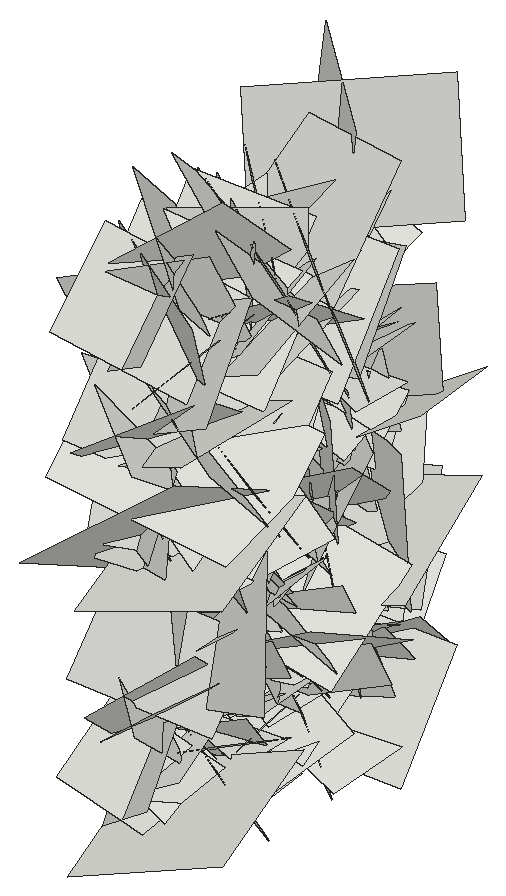
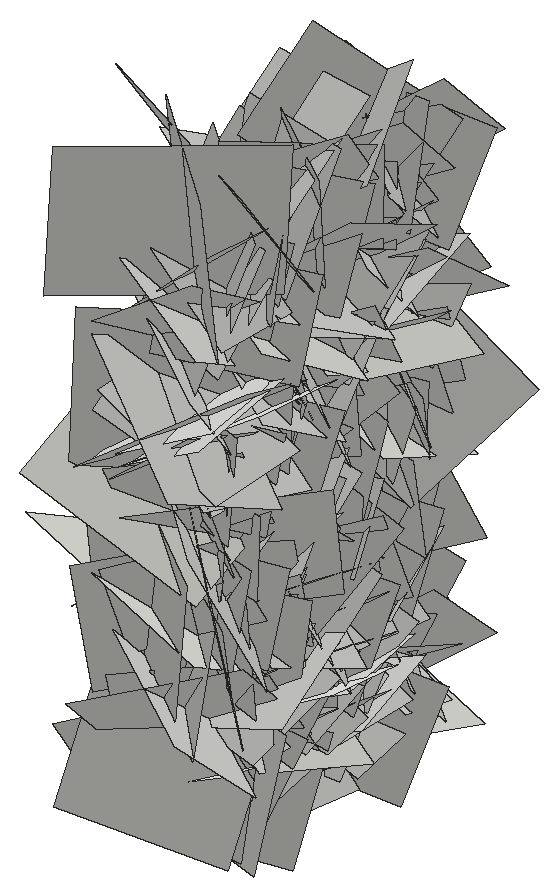
# SketchUp Ruby script. Lengths in inches.
U = 1.inch
M = Sketchup.active_model
def pt(a) = Geom::Point3d.new(a.map { |v| v * U })
def face(e, loops, mat)
  f = e.add_face(loops[0].map { |a| pt(a) })
  loops[1..].each { |l| e.add_face(l.map { |a| pt(a) }).erase! }
  f.material = f.back_material = mat if mat
  f
end
# faces: each face lists its corners as indices into pts; further lists are holes
def faces(e, pts, list, mat = nil) = list.each { |f| face(e, (f[0].is_a?(Array) ? f : [f]).map { |l| l.map { |i| pts[i] } }, mat) }
# xy, xz, yz: faces in a plane at the given z, y or x. An outline is a flat list of corners, or four numbers for a rectangle; further outlines are holes
def ring(l) = l.size == 4 ? [[l[0], l[1]], [l[2], l[1]], [l[2], l[3]], [l[0], l[3]]] : l.each_slice(2).to_a
def flat(e, list, mat, &to3) = list.each { |f| face(e, (f[0].is_a?(Array) ? f : [f]).map { |l| ring(l).map { |u, v| to3.(u, v) } }, mat) }
def xy(e, z, list, mat = nil) = flat(e, list, mat) { |x, y| [x, y, z] }
def xz(e, y, list, mat = nil) = flat(e, list, mat) { |x, z| [x, y, z] }
def yz(e, x, list, mat = nil) = flat(e, list, mat) { |y, z| [x, y, z] }
def lines(e, pts, list) = list.each { |a, b| e.add_line(pt(pts[a]), pt(pts[b])) }
# prism: a flat outline (further loops are holes) pulled along v
def prism(e, loops, v, mat = nil)
  f = face(e, loops, mat); d = Geom::Vector3d.new(v.map { |x| x * U })
  f.pushpull(f.normal.samedirection?(d) ? d.length : -d.length)
end
def box(e, o, s, mat = nil) = prism(e, [[o, [o[0] + s[0], o[1], o[2]], [o[0] + s[0], o[1] + s[1], o[2]], [o[0], o[1] + s[1], o[2]]]], [0, 0, s[2]], mat)
def at(x, y, z, deg = 0) = Geom::Transformation.translation(pt([x, y, z])) * Geom::Transformation.rotation(ORIGIN, Z_AXIS, deg.degrees)
def axes(o, x, y, z) = Geom::Transformation.new([*x, 0, *y, 0, *z, 0, *pt(o).to_a, 1])
def part(name) = M.definitions.add(name)
# library, detail: a bought-in or finely detailed component or shape, given as its bounding box
def library(name, o, s) = part(name).tap { |d| box(d.entities, o, s) }
def detail(e, o, s) = box(e.add_group.entities, o, s)
def put(e, d, t, mat = nil) = e.add_instance(d, t).tap { |i| i.material = mat if mat }
def group(e, t, mat = nil) = e.add_group.tap { |g| g.transformation = t; g.material = mat if mat }.entities
root = M.entities
c1 = part("Component\#6")
p = [[0.01,0,0],[0,3.24,4.54],[4.32,3.24,4.54],[4.33,0,0]]
faces(c1.entities,p,[[0,1,2,3]])
put(root,c1,axes([424.49,166.18,19.56],[0.12535,0.0531,1.28965],[0.2192,1.27754,-0.07157],[-1.35051,0.21229,0.10808]))
put(root,c1,axes([424.49,167.01,8.33],[-0.18631,0.3359,0.73427],[-0.04897,0.74605,-0.35235],[-0.8545,-0.11599,-0.1399]))
put(root,c1,axes([420.52,159.82,10.86],[-0.164,0.05549,-0.7166],[0.119,-0.72215,-0.08015],[0.75252,0.12629,-0.14349]))
put(root,c1,axes([424.49,164.72,6.23],[0.02586,0.29335,1.1723],[0.23754,1.1511,-0.29271],[-1.25874,0.22326,-0.03115]))
put(root,c1,axes([420.52,164.71,11.17],[-0.09162,-0.23701,0.75882],[-0.09076,0.76162,0.22813],[0.83777,0.05659,0.1077]))
put(root,c1,axes([420.52,167.39,12.19],[-0.06725,0.11282,-0.6237],[0.12717,-0.61335,-0.12315],[0.65971,0.12973,-0.03984]))
put(root,c1,axes([420.52,158.25,7.85],[0.01053,0.60228,-0.51533],[-0.19634,-0.49934,-0.58716],[0.81696,-0.12777,-0.13447]))
put(root,c1,axes([424.49,165.51,17.74],[-0.00528,-0.97827,-0.44464],[0.11526,-0.44282,0.97306],[-1.13321,-0.04048,0.10104]))
put(root,c1,axes([424.49,165.75,-1.09],[0.03685,-0.4153,0.96157],[0.02645,0.96216,0.41465],[-1.10996,0.00914,0.04181]))
put(root,c1,axes([424.49,167.74,3.51],[0.11337,-0.86322,0.3774],[-0.28126,0.33685,0.84566],[-0.95821,-0.201,-0.20357]))
put(root,c1,axes([424.49,161.03,4.22],[-0.00206,0.54706,-0.73945],[-0.10036,-0.73565,-0.544],[-0.96983,0.07497,0.05787]))
put(root,c1,axes([424.49,158.84,13.7],[-0.15038,-0.75335,0.50607],[0.08727,0.49942,0.76653],[-0.95804,0.16374,-0.00961]))
put(root,c1,axes([424.49,166.72,20.27],[-0.14718,0.45385,-0.66356],[-0.05291,-0.67695,-0.45256],[-0.85051,-0.03642,0.14299]))
put(root,c1,axes([420.52,158.82,19.64],[0.09205,0.73549,-0.019],[-0.17536,0.00088,-0.72213],[0.75991,-0.08889,-0.16434]))
put(root,c1,axes([424.49,169.09,13.37],[-0.12805,-0.81492,0.2825],[0.01832,0.28292,0.8235],[-0.91406,0.11983,-0.02307]))
put(root,c1,axes([420.52,159.61,12.59],[0.0897,0.16152,-0.57424],[0.01993,-0.58042,-0.16049],[0.632,-0.00462,0.08656]))
put(root,c1,axes([420.52,160.65,18.69],[0.1336,-0.1743,0.59472],[-0.06624,0.60023,0.18916],[0.65357,0.09646,-0.1024]))
put(root,c1,axes([420.52,160.54,14.42],[-0.065,-0.29459,-0.75204],[-0.0763,-0.74921,0.29935],[0.85274,-0.0895,-0.03054]))
put(root,c1,axes([420.52,161.26,10.83],[-0.08958,0.45503,-0.59155],[0.06652,-0.58889,-0.46195],[0.78829,0.10141,-0.02824]))
put(root,c1,axes([424.49,170.16,13.55],[0.14984,-1.04824,-0.22204],[-0.00627,-0.22472,1.05715],[-1.13577,-0.13705,-0.03513]))
put(root,c1,axes([420.52,160.97,6.7],[0.04912,0.73058,0.10133],[-0.09877,0.10652,-0.72536],[0.77557,-0.03271,-0.0988]))
put(root,c1,axes([424.49,163.26,10.51],[-0.09772,0.8385,-0.3881],[0.10419,-0.37892,-0.842],[-0.97385,-0.12468,-0.05114]))
put(root,c1,axes([420.52,159.79,25.07],[-0.1328,0.69586,-0.68383],[-0.18687,-0.69425,-0.67416],[1.01714,-0.03669,-0.21313]))
put(root,c1,axes([424.49,167.39,3.05],[0.22625,-1.02118,-0.283],[-0.12014,-0.30902,1.02962],[-1.11681,-0.17363,-0.16809]))
put(root,c1,axes([420.52,159.32,12.84],[0.06752,-0.16321,-0.59207],[0.0871,-0.58763,0.17083],[0.64514,0.09641,0.0389]))
put(root,c1,axes([424.49,166.22,16.78],[0.0558,0.90138,-0.08554],[-0.09664,-0.07998,-0.89882],[-0.95488,0.06076,0.08597]))
put(root,c1,axes([420.52,166.8,6.58],[-0.19077,-0.84984,-0.315],[0.00737,-0.32244,0.86593],[0.9607,-0.16629,-0.0692]))
put(root,c1,axes([424.49,159.03,23.29],[0.13252,0.38295,-0.87838],[-0.10893,-0.87536,-0.39626],[-1.00987,0.14467,-0.07253]))
put(root,c1,axes([420.52,160.57,3.12],[0.03509,0.82869,0.13415],[-0.15764,0.13792,-0.81528],[0.87577,-0.00838,-0.15213]))
put(root,c1,axes([420.52,164.04,15.7],[0.03624,-0.6234,-0.24842],[0.08,-0.24359,0.62167],[0.70683,0.05954,-0.05762]))
put(root,c1,axes([424.49,170.98,12.21],[0.31631,-0.51758,-1.19288],[0.16648,-1.20059,0.56021],[-1.36826,-0.26573,-0.20761]))
put(root,c1,axes([420.52,169.83,13.22],[0.13817,-0.64015,-0.16037],[-0.03989,-0.17041,0.64965],[0.69839,0.11692,0.06883]))
put(root,c1,axes([420.52,161.46,7.67],[0.11157,-0.00104,0.59962],[0.09459,0.60203,-0.01462],[0.62852,-0.09042,-0.10424]))
put(root,c1,axes([424.49,168.08,9.41],[0.11593,0.02752,-0.90523],[-0.14705,-0.90054,-0.04413],[-0.94866,0.14295,-0.10378]))
put(root,c1,axes([420.52,169.26,18.83],[0.02849,-0.83115,-0.05333],[-0.13283,-0.05679,0.82186],[0.87278,0.01849,0.12683]))
put(root,c1,axes([420.52,165.55,15.88],[-0.02597,-0.35934,-0.67832],[0.02345,-0.67872,0.35875],[0.81334,0.00809,-0.032]))
put(root,c1,axes([420.52,167.12,21.5],[0.0656,0.35319,-0.61189],[0.00255,-0.61434,-0.35436],[0.7489,-0.02885,0.0548]))
put(root,c1,axes([424.49,164.04,2.37],[0.08884,-0.86849,0.07962],[-0.14736,0.06566,0.86256],[-0.91264,-0.09515,-0.13152]))
put(root,c1,axes([424.49,162.54,0.74],[0.05881,-0.79857,0.25436],[-0.14334,0.24305,0.79255],[-0.87675,-0.0933,-0.11251]))
put(root,c1,axes([424.49,157.37,3.29],[-0.12325,0.67494,0.21472],[-0.06797,0.20667,-0.68436],[-0.74769,-0.13004,0.02682]))
put(root,c1,axes([424.49,166.02,4.84],[0.16866,0.71959,0.68076],[-0.0323,0.69272,-0.72511],[-1.04952,0.09433,0.13172]))
put(root,c1,axes([420.52,162.4,12.14],[0.15913,-0.1111,0.71617],[-0.10617,0.72117,0.13287],[0.76084,0.12387,-0.13124]))
put(root,c1,axes([420.52,165.06,16.01],[-0.24936,0.99659,0.4051],[-0.07669,0.39908,-1.02378],[1.13774,0.24532,0.01978]))
put(root,c1,axes([420.52,164.7,6.68],[-0.19863,-0.78204,0.62344],[-0.03401,0.63866,0.7915],[1.0596,-0.1261,0.14227]))
put(root,c1,axes([424.49,166.67,11.65],[-0.03639,0.32382,0.70516],[-0.0632,0.70266,-0.32558],[-0.82009,-0.06852,-0.0062]))
put(root,c1,axes([424.49,166.25,3.34],[-0.10377,-0.78092,-0.09398],[0.04515,-0.09983,0.78516],[-0.83253,0.09192,0.05429]))
put(root,c1,axes([424.49,167.84,10.46],[0.01526,0.23241,-0.73689],[-0.14958,-0.72384,-0.23105],[-0.80526,0.13886,0.02896]))
put(root,c1,axes([424.49,164.66,7.18],[0.03191,0.54978,-0.59147],[-0.106,-0.58478,-0.54866],[-0.84939,0.09364,0.04625]))
put(root,c1,axes([424.49,155.24,20.59],[-0.01301,0.69003,0.71111],[0.211,0.69839,-0.67424],[-1.02891,0.13449,-0.14726]))
put(root,c1,axes([424.49,167.39,19.82],[-0.12929,0.6108,0.35138],[-0.02449,0.35295,-0.62154],[-0.74654,-0.11736,-0.04046]))
put(root,c1,axes([420.52,165.07,9.38],[0.13081,0.27606,-0.70722],[-0.08788,-0.70731,-0.29057],[0.79993,-0.12284,0.08373]))
put(root,c1,axes([424.49,159.79,6],[0.13547,0.51146,0.93772],[0.15367,0.92736,-0.52557],[-1.12174,0.18881,0.04125]))
put(root,c1,axes([424.49,159.9,13.67],[0.02397,0.44215,0.82689],[0.11898,0.8199,-0.44149],[-0.98679,0.1096,-0.03314]))
put(root,c1,axes([420.52,164.44,22.83],[-0.02931,-0.02413,-0.88007],[-0.04764,-0.87932,0.02552],[0.93201,-0.0457,-0.02637]))
put(root,c1,axes([424.49,168.54,15.47],[0.051,0.16682,-0.79913],[-0.09039,-0.79511,-0.17112],[-0.86061,0.0934,-0.02938]))
put(root,c1,axes([424.49,155.625,2.89],[-0.13104,0.56412,0.5606],[0.11872,0.57403,-0.55293],[-0.83462,-0.00692,-0.16667]))
put(root,c1,axes([424.49,163.43,17.5],[0.07736,-0.30856,0.98844],[0.18729,0.98007,0.2929],[-1.08152,0.14765,0.12143]))
put(root,c1,axes([420.52,163.43,17.5],[-0.07736,-0.30856,0.98844],[-0.18729,0.98007,0.2929],[1.08152,0.14765,0.12143]))
put(root,c1,axes([420.52,155.625,2.89],[0.13104,0.56412,0.5606],[-0.11872,0.57403,-0.55293],[0.83462,-0.00692,-0.16667]))
put(root,c1,axes([420.52,168.54,15.47],[-0.051,0.16682,-0.79913],[0.09039,-0.79511,-0.17112],[0.86061,0.0934,-0.02938]))
put(root,c1,axes([424.49,164.44,22.83],[0.02931,-0.02413,-0.88007],[0.04764,-0.87932,0.02552],[-0.93201,-0.0457,-0.02637]))
put(root,c1,axes([420.52,159.9,13.67],[-0.02397,0.44215,0.82689],[-0.11898,0.8199,-0.44149],[0.98679,0.1096,-0.03314]))
put(root,c1,axes([420.52,159.79,6],[-0.13547,0.51146,0.93772],[-0.15367,0.92736,-0.52557],[1.12174,0.18881,0.04125]))
put(root,c1,axes([424.49,165.07,9.38],[-0.13081,0.27606,-0.70722],[0.08788,-0.70731,-0.29057],[-0.79993,-0.12284,0.08373]))
put(root,c1,axes([420.52,167.39,19.82],[0.12929,0.6108,0.35138],[0.02449,0.35295,-0.62154],[0.74654,-0.11736,-0.04046]))
put(root,c1,axes([420.52,155.24,20.59],[0.01301,0.69003,0.71111],[-0.211,0.69839,-0.67424],[1.02891,0.13449,-0.14726]))
put(root,c1,axes([420.52,164.66,7.18],[-0.03191,0.54978,-0.59147],[0.106,-0.58478,-0.54866],[0.84939,0.09364,0.04625]))
put(root,c1,axes([420.52,167.84,10.46],[-0.01526,0.23241,-0.73689],[0.14958,-0.72384,-0.23105],[0.80526,0.13886,0.02896]))
put(root,c1,axes([420.52,166.25,3.34],[0.10377,-0.78092,-0.09398],[-0.04515,-0.09983,0.78516],[0.83253,0.09192,0.05429]))
put(root,c1,axes([420.52,166.67,11.65],[0.03639,0.32382,0.70516],[0.0632,0.70266,-0.32558],[0.82009,-0.06852,-0.0062]))
put(root,c1,axes([424.49,164.7,6.68],[0.19863,-0.78204,0.62344],[0.03401,0.63866,0.7915],[-1.0596,-0.1261,0.14227]))
put(root,c1,axes([424.49,165.06,16.01],[0.24936,0.99659,0.4051],[0.07669,0.39908,-1.02378],[-1.13774,0.24532,0.01978]))
put(root,c1,axes([424.49,162.4,12.14],[-0.15913,-0.1111,0.71617],[0.10617,0.72117,0.13287],[-0.76084,0.12387,-0.13124]))
put(root,c1,axes([420.52,166.02,4.84],[-0.16866,0.71959,0.68076],[0.0323,0.69272,-0.72511],[1.04952,0.09433,0.13172]))
put(root,c1,axes([420.52,157.37,3.29],[0.12325,0.67494,0.21472],[0.06797,0.20667,-0.68436],[0.74769,-0.13004,0.02682]))
put(root,c1,axes([420.52,162.54,0.74],[-0.05881,-0.79857,0.25436],[0.14334,0.24305,0.79255],[0.87675,-0.0933,-0.11251]))
put(root,c1,axes([420.52,164.04,2.37],[-0.08884,-0.86849,0.07962],[0.14736,0.06566,0.86256],[0.91264,-0.09515,-0.13152]))
put(root,c1,axes([424.49,167.12,21.5],[-0.0656,0.35319,-0.61189],[-0.00255,-0.61434,-0.35436],[-0.7489,-0.02885,0.0548]))
put(root,c1,axes([424.49,165.55,15.88],[0.02597,-0.35934,-0.67832],[-0.02345,-0.67872,0.35875],[-0.81334,0.00809,-0.032]))
put(root,c1,axes([424.49,169.26,18.83],[-0.02849,-0.83115,-0.05333],[0.13283,-0.05679,0.82186],[-0.87278,0.01849,0.12683]))
put(root,c1,axes([420.52,168.08,9.41],[-0.11593,0.02752,-0.90523],[0.14705,-0.90054,-0.04413],[0.94866,0.14295,-0.10378]))
put(root,c1,axes([424.49,161.46,7.67],[-0.11157,-0.00104,0.59962],[-0.09459,0.60203,-0.01462],[-0.62852,-0.09042,-0.10424]))
put(root,c1,axes([424.49,169.83,13.22],[-0.13817,-0.64015,-0.16037],[0.03989,-0.17041,0.64965],[-0.69839,0.11692,0.06883]))
put(root,c1,axes([420.52,170.98,12.21],[-0.31631,-0.51758,-1.19288],[-0.16648,-1.20059,0.56021],[1.36826,-0.26573,-0.20761]))
put(root,c1,axes([424.49,164.04,15.7],[-0.03624,-0.6234,-0.24842],[-0.08,-0.24359,0.62167],[-0.70683,0.05954,-0.05762]))
put(root,c1,axes([424.49,160.57,3.12],[-0.03509,0.82869,0.13415],[0.15764,0.13792,-0.81528],[-0.87577,-0.00838,-0.15213]))
put(root,c1,axes([420.52,159.03,23.29],[-0.13252,0.38295,-0.87838],[0.10893,-0.87536,-0.39626],[1.00987,0.14467,-0.07253]))
put(root,c1,axes([424.49,166.8,6.58],[0.19077,-0.84984,-0.315],[-0.00737,-0.32244,0.86593],[-0.9607,-0.16629,-0.0692]))
put(root,c1,axes([420.52,166.22,16.78],[-0.0558,0.90138,-0.08554],[0.09664,-0.07998,-0.89882],[0.95488,0.06076,0.08597]))
put(root,c1,axes([424.49,159.32,12.84],[-0.06752,-0.16321,-0.59207],[-0.0871,-0.58763,0.17083],[-0.64514,0.09641,0.0389]))
put(root,c1,axes([420.52,167.39,3.05],[-0.22625,-1.02118,-0.283],[0.12014,-0.30902,1.02962],[1.11681,-0.17363,-0.16809]))
put(root,c1,axes([424.49,159.79,25.07],[0.1328,0.69586,-0.68383],[0.18687,-0.69425,-0.67416],[-1.01714,-0.03669,-0.21313]))
put(root,c1,axes([420.52,163.26,10.51],[0.09772,0.8385,-0.3881],[-0.10419,-0.37892,-0.842],[0.97385,-0.12468,-0.05114]))
put(root,c1,axes([424.49,160.97,6.7],[-0.04912,0.73058,0.10133],[0.09877,0.10652,-0.72536],[-0.77557,-0.03271,-0.0988]))
put(root,c1,axes([420.52,170.16,13.55],[-0.14984,-1.04824,-0.22204],[0.00627,-0.22472,1.05715],[1.13577,-0.13705,-0.03513]))
put(root,c1,axes([424.49,161.26,10.83],[0.08958,0.45503,-0.59155],[-0.06652,-0.58889,-0.46195],[-0.78829,0.10141,-0.02824]))
put(root,c1,axes([424.49,160.54,14.42],[0.065,-0.29459,-0.75204],[0.0763,-0.74921,0.29935],[-0.85274,-0.0895,-0.03054]))
put(root,c1,axes([424.49,160.65,18.69],[-0.1336,-0.1743,0.59472],[0.06624,0.60023,0.18916],[-0.65357,0.09646,-0.1024]))
put(root,c1,axes([424.49,159.61,12.59],[-0.0897,0.16152,-0.57424],[-0.01993,-0.58042,-0.16049],[-0.632,-0.00462,0.08656]))
put(root,c1,axes([420.52,169.09,13.37],[0.12805,-0.81492,0.2825],[-0.01832,0.28292,0.8235],[0.91406,0.11983,-0.02307]))
put(root,c1,axes([424.49,158.82,19.64],[-0.09205,0.73549,-0.019],[0.17536,0.00088,-0.72213],[-0.75991,-0.08889,-0.16434]))
put(root,c1,axes([420.52,166.72,20.27],[0.14718,0.45385,-0.66356],[0.05291,-0.67695,-0.45256],[0.85051,-0.03642,0.14299]))
put(root,c1,axes([420.52,158.84,13.7],[0.15038,-0.75335,0.50607],[-0.08727,0.49942,0.76653],[0.95804,0.16374,-0.00961]))
put(root,c1,axes([420.52,161.03,4.22],[0.00206,0.54706,-0.73945],[0.10036,-0.73565,-0.544],[0.96983,0.07497,0.05787]))
put(root,c1,axes([420.52,167.74,3.51],[-0.11337,-0.86322,0.3774],[0.28126,0.33685,0.84566],[0.95821,-0.201,-0.20357]))
put(root,c1,axes([420.52,165.75,-1.09],[-0.03685,-0.4153,0.96157],[-0.02645,0.96216,0.41465],[1.10996,0.00914,0.04181]))
put(root,c1,axes([420.52,165.51,17.74],[0.00528,-0.97827,-0.44464],[-0.11526,-0.44282,0.97306],[1.13321,-0.04048,0.10104]))
put(root,c1,axes([424.49,158.25,7.85],[-0.01053,0.60228,-0.51533],[0.19634,-0.49934,-0.58716],[-0.81696,-0.12777,-0.13447]))
put(root,c1,axes([424.49,167.39,12.19],[0.06725,0.11282,-0.6237],[-0.12717,-0.61335,-0.12315],[-0.65971,0.12973,-0.03984]))
put(root,c1,axes([424.49,164.71,11.17],[0.09162,-0.23701,0.75882],[0.09076,0.76162,0.22813],[-0.83777,0.05659,0.1077]))
put(root,c1,axes([420.52,164.72,6.23],[-0.02586,0.29335,1.1723],[-0.23754,1.1511,-0.29271],[1.25874,0.22326,-0.03115]))
put(root,c1,axes([424.49,159.82,10.86],[0.164,0.05549,-0.7166],[-0.119,-0.72215,-0.08015],[-0.75252,0.12629,-0.14349]))
put(root,c1,axes([420.52,167.01,8.33],[0.18631,0.3359,0.73427],[0.04897,0.74605,-0.35235],[0.8545,-0.11599,-0.1399]))
put(root,c1,axes([420.52,166.18,19.56],[-0.12535,0.0531,1.28965],[-0.2192,1.27754,-0.07157],[1.35051,0.21229,0.10808]))
put(root,c1,axes([420.52,168.14,0.12],[-0.06773,-0.63363,0.78179],[0.11595,0.77435,0.63654],[1.06038,-0.12515,-0.01967]))
put(root,c1,axes([420.52,169.19,10.7],[-0.0913,0.46499,-1.24639],[-0.29576,-1.22753,-0.43867],[1.37875,-0.23253,-0.17663]))
put(root,c1,axes([424.49,165.96,10.85],[0.09912,0.20412,-0.70693],[0.02587,-0.71308,-0.20267],[-0.77953,0.00229,-0.09661]))
put(root,c1,axes([424.49,161.25,17.66],[0.25985,0.898,-0.37026],[0.14737,-0.41038,-0.90325],[-1.01902,0.16964,-0.22504]))
put(root,c1,axes([424.49,162.79,15.86],[0.07285,0.46729,0.4905],[-0.02436,0.49435,-0.46773],[-0.71769,0.03066,0.06566]))
put(root,c1,axes([420.52,167.22,15.375],[-0.0235,-0.92066,-0.53568],[-0.01768,-0.53543,0.92093],[1.12894,-0.02755,0.00327]))
put(root,c1,axes([420.52,167.28,17.92],[-0.19972,-0.96368,-0.57877],[0.14667,-0.60226,0.95775],[1.18251,-0.08806,-0.21655]))
put(root,c1,axes([420.52,157.18,19.73],[-0.07599,0.81527,0.8297],[-0.084,0.82592,-0.8184],[1.23014,0.10676,-0.00463]))
put(root,c1,axes([420.52,167.18,1.59],[-0.07507,-1.0991,0.32301],[-0.05871,0.32653,1.09895],[1.2129,-0.05222,0.07319]))
put(root,c1,axes([420.52,168.87,14.79],[0.03205,0.06087,-1.12787],[-0.16204,-1.11767,-0.06442],[1.18627,-0.15431,0.02167]))
put(root,c1,axes([420.52,166.01,11.8],[0.21466,0.53877,-0.68228],[-0.03009,-0.69607,-0.55809],[0.92102,-0.14831,0.14079]))
put(root,c1,axes([420.52,163.57,3.71],[0.11292,-0.2033,0.99476],[-0.09749,0.99417,0.21302],[1.07181,0.11185,-0.08542]))
put(root,c1,axes([420.52,159.91,9.22],[-0.2022,-1.20502,0.50539],[-0.1049,0.52261,1.20871],[1.38114,-0.13672,0.1658]))
put(root,c1,axes([420.52,162.44,14.8125],[-0.22172,-1.13603,-0.19278],[0.19013,-0.22565,1.13507],[1.20652,-0.17321,-0.21429]))
put(root,c1,axes([420.52,160.62,5.12],[0.08568,1.04485,0.18773],[-0.09569,0.19436,-1.04286],[1.1212,-0.06325,-0.10335]))
put(root,c1,axes([424.49,162.91,7.6875],[0.03517,0.6334,0.29771],[0.1292,0.28826,-0.62688],[-0.73053,0.08147,-0.09654]))
put(root,c1,axes([420.52,163.93,5.47],[0.11462,-1.01834,-0.26907],[-0.10191,-0.2789,1.0169],[1.11183,0.07941,0.12095]))
put(root,c1,axes([420.52,156.14,6.5],[0.17845,0.35117,0.84391],[0.01887,0.85668,-0.36003],[0.96872,-0.08137,-0.14844]))
put(root,c1,axes([424.49,170.02,6.34],[0.13634,-0.30577,-0.6303],[0.02329,-0.63876,0.31436],[-0.74222,-0.07621,-0.10592]))
put(root,c1,axes([420.52,160.14,4.78],[0.03826,-0.47304,0.81506],[0.18962,0.80427,0.45886],[0.98077,-0.13704,-0.12051]))
put(root,c1,axes([420.52,166.625,12.7],[0.17127,1.04033,-0.10676],[-0.13463,-0.08771,-1.04688],[1.10034,-0.17266,-0.11147]))
put(root,c1,axes([420.52,168.99,0.33],[0.20008,-0.71049,0.66963],[-0.07161,0.67089,0.73087],[1.03242,0.18422,-0.07908]))
put(root,c1,axes([420.52,164.18,5.53],[0.00871,-1.21515,-0.1589],[-0.11926,-0.15898,1.20995],[1.29354,-0.00648,0.11262]))
put(root,c1,axes([424.49,159.77,13.93],[0.14822,0.47929,0.38572],[-0.01533,0.39801,-0.48932],[-0.65196,0.0996,0.0992]))
put(root,c1,axes([420.52,165.6875,8.33],[0.14254,-0.77018,0.64298],[0.05856,0.65343,0.77114],[1.06187,0.06735,-0.12884]))
put(root,c1,axes([420.52,164.53,2.65],[0.11418,0.95876,0.15487],[0.16789,0.13639,-0.95453],[1.01568,-0.13033,0.14037]))
put(root,c1,axes([424.49,155.94,6.59],[0.14653,0.65267,0.04592],[0.0729,0.03218,-0.6644],[-0.6897,0.14207,-0.06047]))
put(root,c1,axes([420.52,170.79,17.67],[0.07972,-0.69903,-0.88266],[-0.01234,-0.88506,0.69994],[1.19343,0.03754,0.0662]))
put(root,c1,axes([420.52,165.97,13.03],[0.11695,-0.23373,1.15092],[-0.10796,1.14973,0.24325],[1.24018,0.12213,-0.08736]))
put(root,c1,axes([424.49,164.09,3.1],[0.16189,-0.51758,0.36968],[0.06161,0.38995,0.52196],[-0.67139,-0.08902,0.13704]))
put(root,c1,axes([420.52,155.93,16.01],[0.06166,0.77521,1.08886],[-0.24821,1.07895,-0.75564],[1.39492,0.15772,-0.18259]))
put(root,c1,axes([420.52,163.21,2.24],[-0.08398,-0.53221,1.10764],[0.11648,1.10243,0.53756],[1.29738,-0.13342,0.02343]))
put(root,c1,axes([420.52,161.02,12.77],[0.04866,0.36936,-1.04237],[0.12613,-1.03886,-0.36288],[1.16543,0.09701,0.0828]))
put(root,c1,axes([420.52,162.03,18.62],[0.15865,-0.78055,-0.79386],[-0.03617,-0.80384,0.78393],[1.17956,0.08034,0.13081]))
put(root,c1,axes([420.52,161.03,16.77],[-0.02327,0.73455,-0.90907],[0.17416,-0.89826,-0.72978],[1.22657,0.14148,0.08637]))
put(root,c1,axes([420.52,163.86,1.73],[0.03729,0.66749,1.03354],[-0.00972,1.03407,-0.66752],[1.30413,-0.01138,-0.03452]))
put(root,c1,axes([420.52,162.85,15.75],[0.04254,-1.00522,0.67204],[0.02385,0.67292,1.00519],[1.28151,0.02084,-0.04102]))
put(root,c1,axes([420.52,163.36,23.49],[0.04873,0.57368,-1.00395],[0.12423,-1.00188,-0.56714],[1.21936,0.07915,0.09791]))
put(root,c1,axes([420.52,159.69,18.96],[0.02704,0.74145,1.09535],[-0.09362,1.09406,-0.73853],[1.39894,0.05888,-0.07059]))
put(root,c1,axes([420.52,166.4,18.65],[-0.092,-1.19571,-0.63762],[0.0325,-0.6405,1.19693],[1.43603,-0.06211,-0.06794]))
put(root,c1,axes([420.52,155.03,14.95],[-0.10989,1.07322,0.82249],[0.07177,0.82799,-1.07186],[1.43147,0.04087,0.11688]))
put(root,c1,axes([420.52,159.14,18.38],[0.07521,0.79304,-0.86536],[0.12573,-0.86735,-0.78513],[1.23784,0.03991,0.13233]))
put(root,c1,axes([420.52,168.375,23.9],[-0.0952,-0.72561,-1.04974],[0.29336,-1.03837,0.69407],[1.32049,0.17837,-0.22987]))
put(root,c1,axes([420.52,157.93,15.34],[0.27083,1.19165,0.15594],[-0.0802,0.17506,-1.21378],[1.27139,-0.2428,-0.10978]))
put(root,c1,axes([420.52,162.31,11.53],[0.17206,0.75955,-0.87532],[0.12131,-0.89005,-0.75111],[1.22246,-0.01858,0.19774]))
put(root,c1,axes([420.52,165.1,2.71],[-0.06092,-1.21711,0.58199],[0.18306,0.57109,1.21136],[1.41828,-0.12599,-0.13136]))
put(root,c1,axes([420.52,170.58,10.37],[0.24309,-1.14649,0.14454],[0.04952,0.15643,1.16674],[1.2239,0.22139,-0.07591]))
put(root,c1,axes([420.52,161.07,7.88],[0.0926,0.91308,0.78861],[0.24837,0.76278,-0.90913],[1.25453,-0.21841,0.12178]))
put(root,c1,axes([420.52,171.01,11.29],[0.23144,-0.15428,-1.27652],[-0.01824,-1.29503,0.15357],[1.36284,0.00887,0.21884]))
put(root,c1,axes([420.52,167.61,21.95],[0.32344,0.31012,-1.26322],[-0.1451,-1.28265,-0.34796],[1.37111,-0.2089,0.26116]))
put(root,c1,axes([420.52,161.91,24.73],[0.20116,0.87735,-0.9177],[0.06395,-0.93308,-0.87958],[1.34427,-0.0869,0.17917]))
put(root,c1,axes([420.52,161.24,11.55],[0.08722,-1.18104,-0.51149],[0.30261,-0.48302,1.16122],[1.33028,0.18731,-0.23062]))
put(root,c1,axes([420.52,160.65,1.35],[0.1594,-1.22011,-0.46707],[0.28659,-0.43091,1.2127],[1.35486,0.2347,-0.20157]))
put(root,c1,axes([420.52,170.67,8.29],[0.13658,-1.14766,-0.62909],[0.33753,-0.58565,1.13362],[1.34561,0.26339,-0.2205]))
put(root,c1,axes([420.52,161.87,9.58],[0.35888,-0.49511,-1.17449],[0.11741,-1.19919,0.53746],[1.34594,0.23663,0.26628]))
